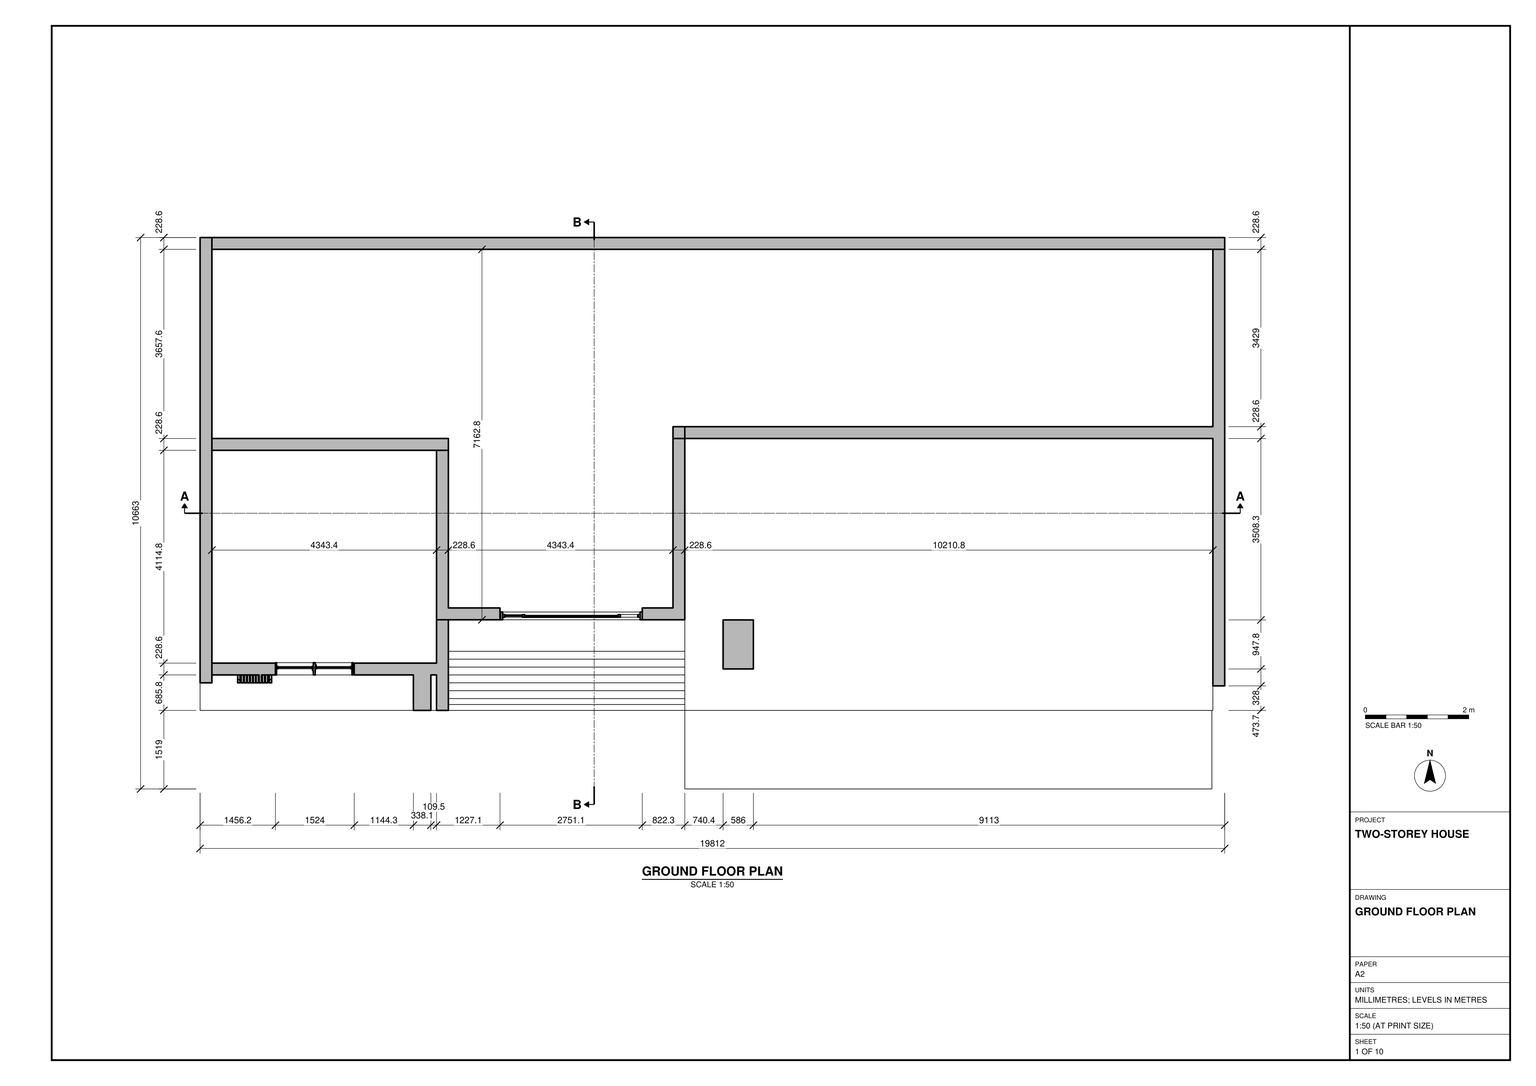
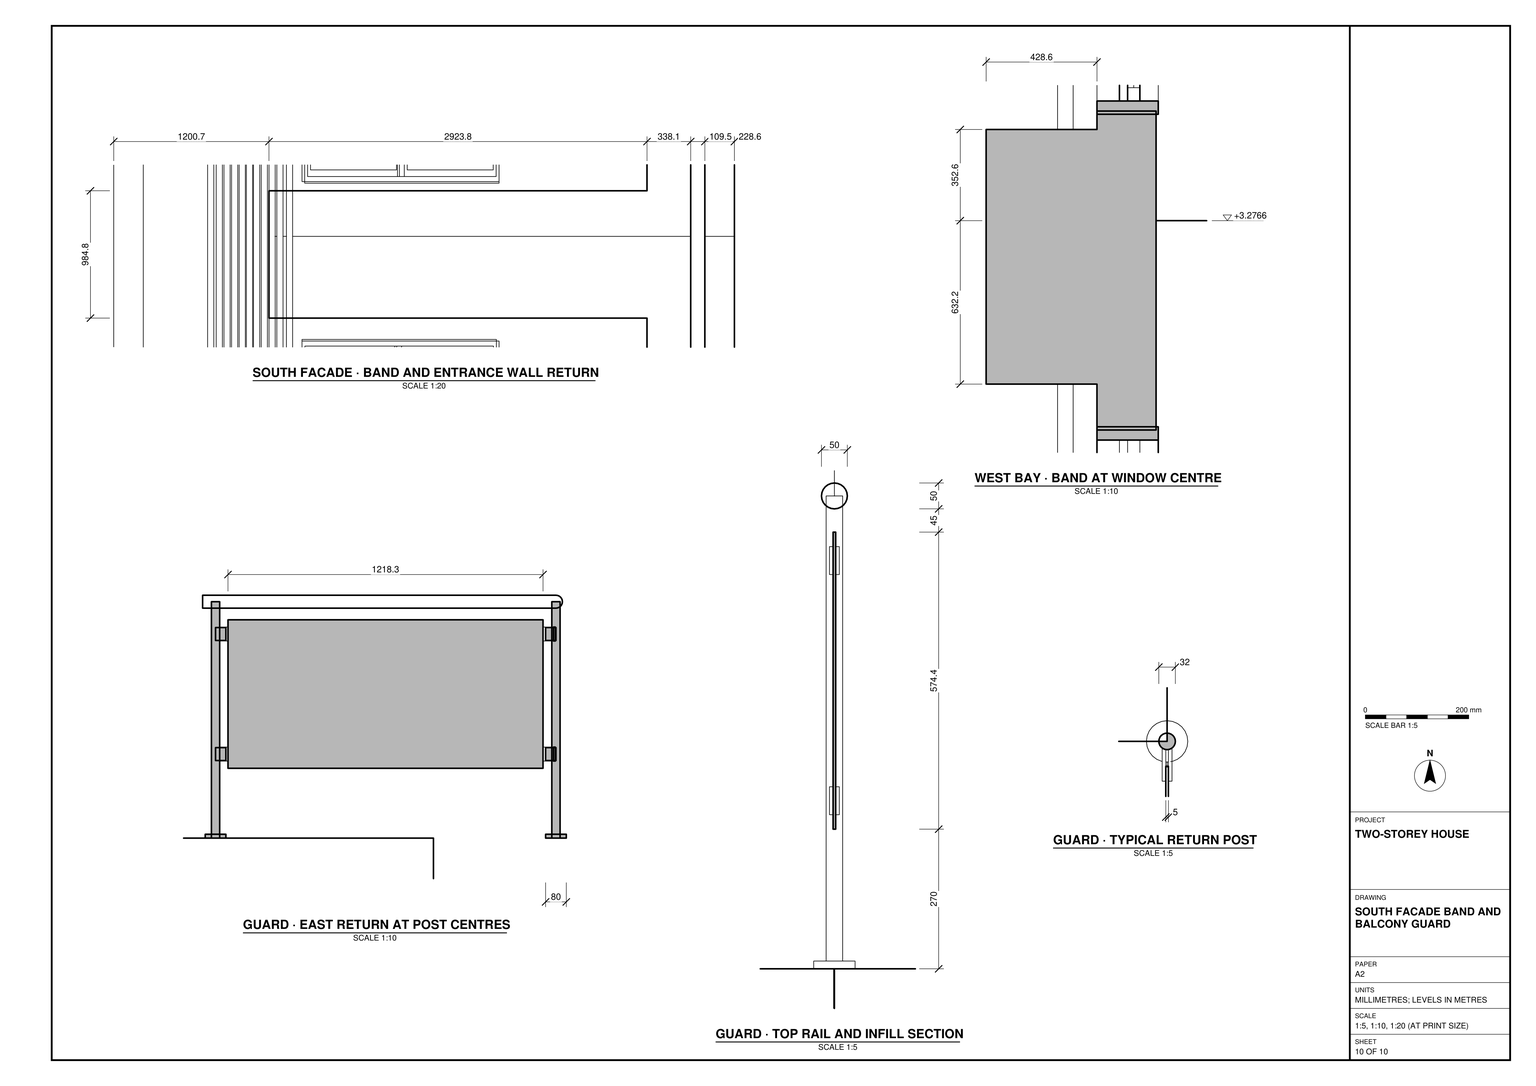
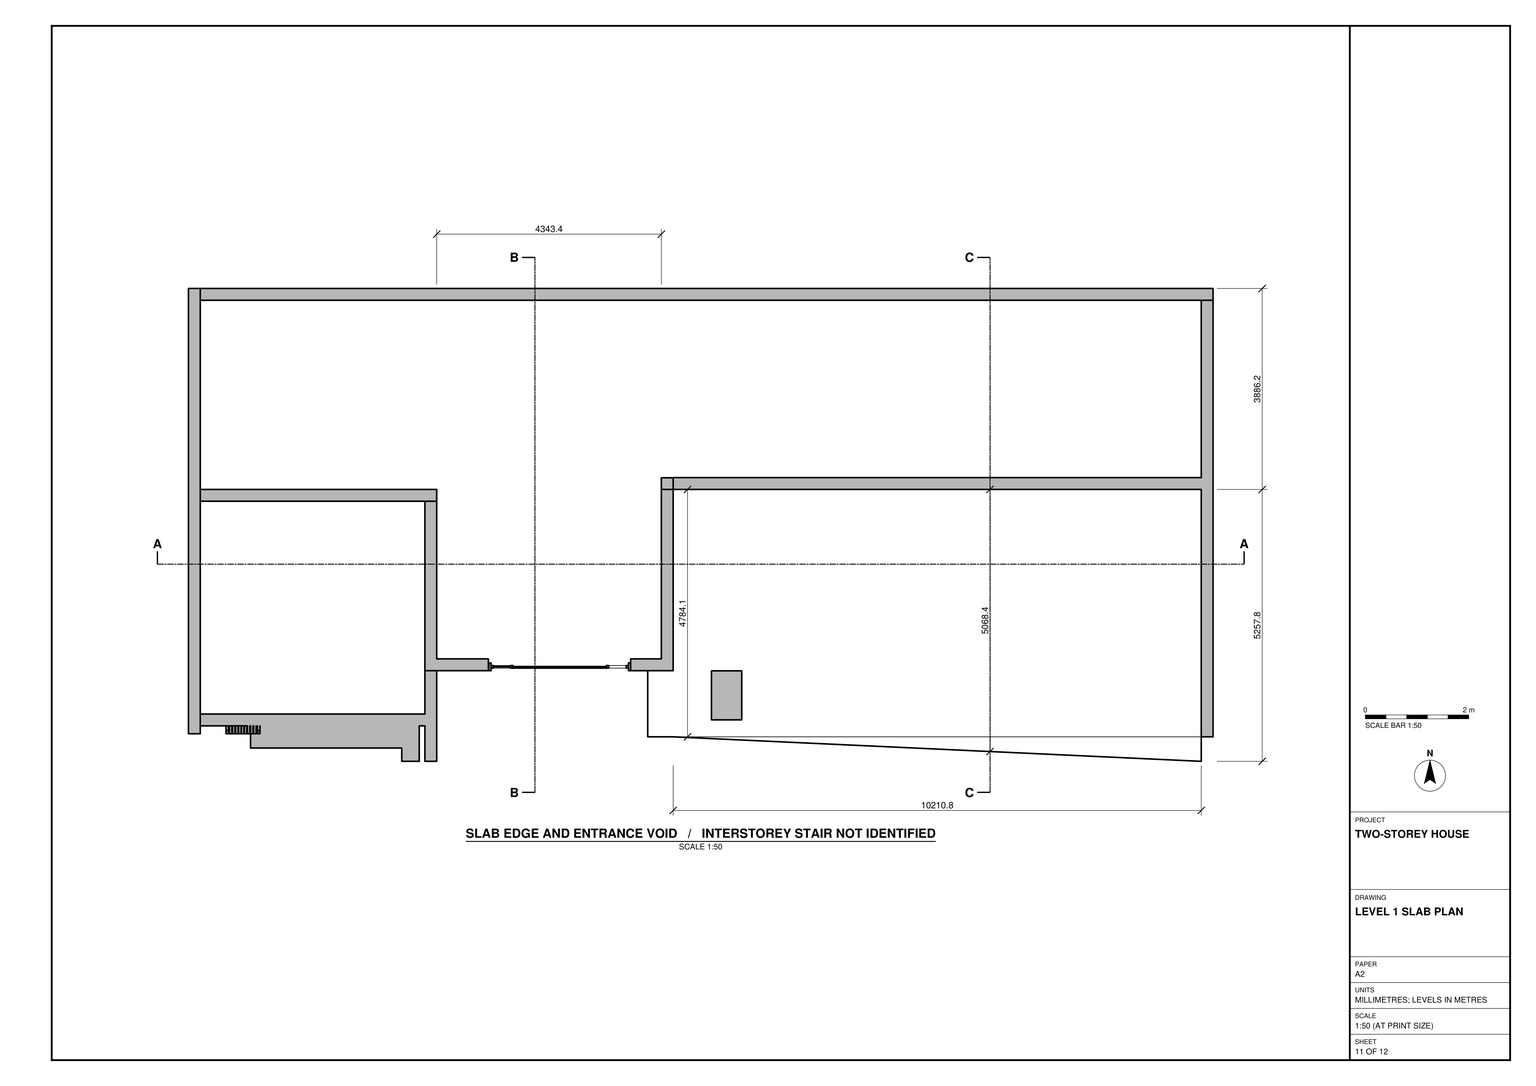
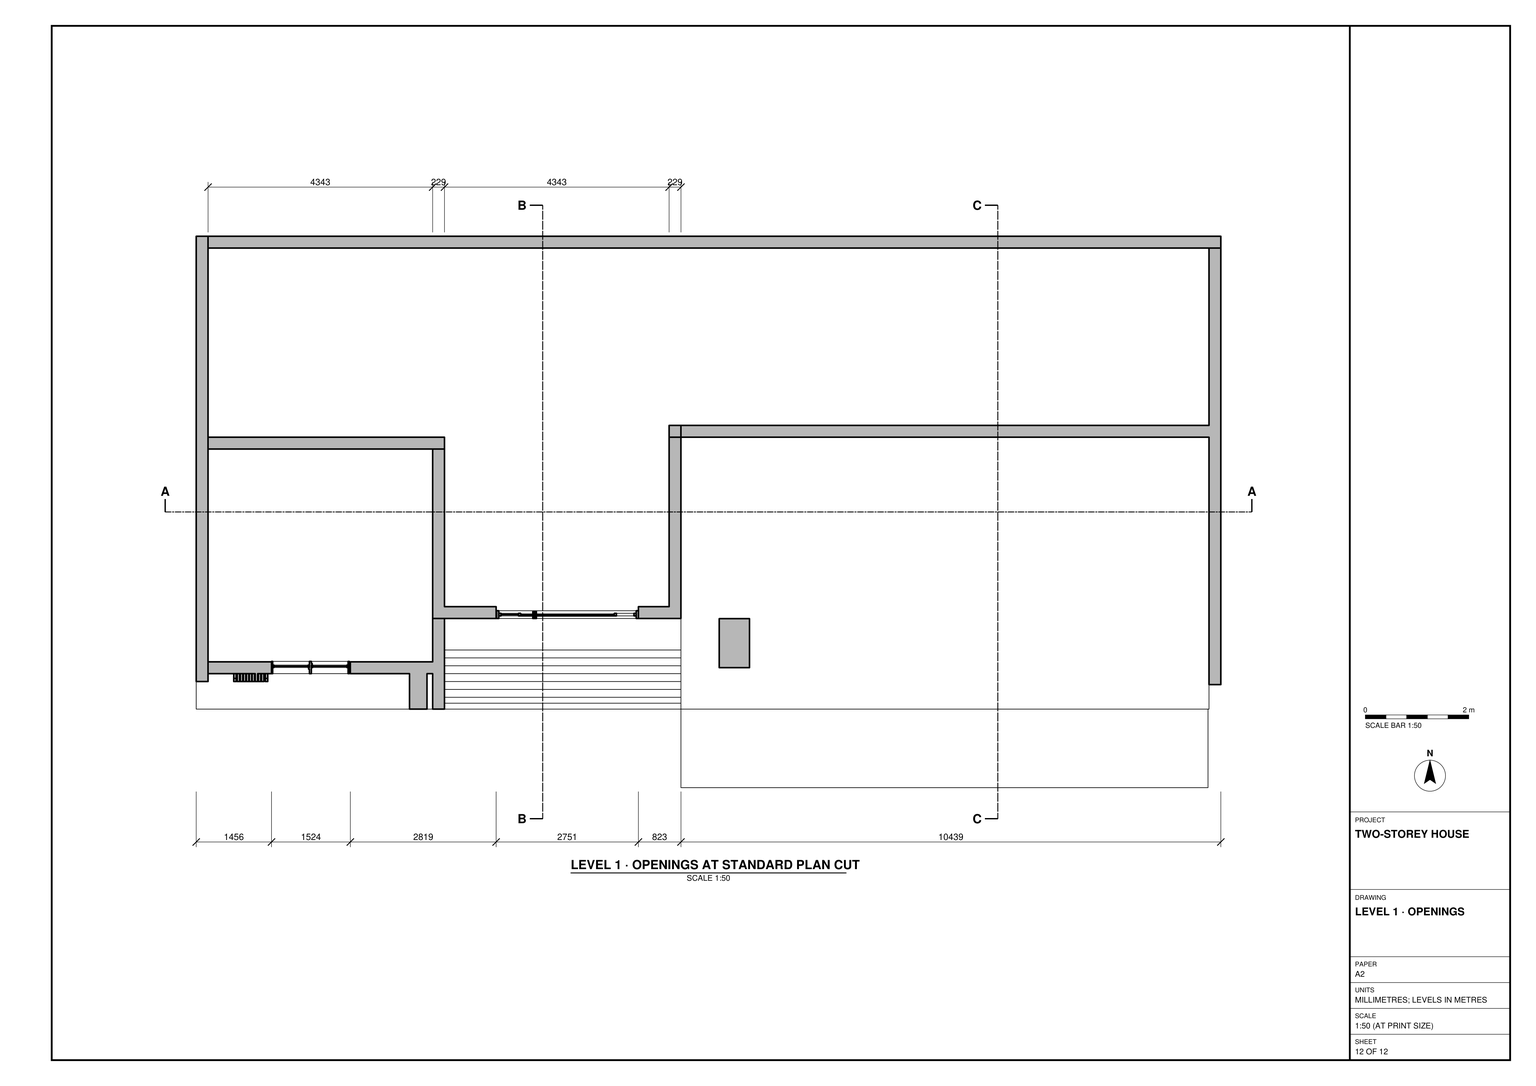
Build the house in SketchUp from task_files/diagram_01.pdf. Work in millimetres and orient the plan with the entrance on the south side. The overall model is 19812 mm wide from west to east, 10663.2 mm deep from north to south and 8074 mm high. Set the ground floor at 0 mm and the upper floor at +3276.6 mm.

Lay out the continuous north wall, the west bay, the central entrance bay and the wider east bay. Use the wall thicknesses shown, including the walls dimensioned at 228.6 mm. Fit the door and window units into their openings. Run the exterior steps across the central bay up to the entrance and place the rectangular pier to their east.

Use the slab plan to shape the upper floor around the entrance void and to set out the angled balcony edge over the east bay. Follow the sheets for the roof profile. Model the projecting horizontal band on the west bay where it meets the entrance wall return. Use the guard details to place the balcony posts, top rail and raised infill panels, including the return at the east end.

Include built-in joinery and main furniture only where shown. Decor and loose items may be any suitable library components. Keep the walls, slabs, roof and each furniture or joinery piece in separate groups or components, and use components for repeated parts. Save one SketchUp model as output_files/two_storey_house_with_a_recessed_entrance_and_balcony.skp.

# SketchUp Ruby script. Lengths in millimetres.
U = 1.mm
M = Sketchup.active_model
def pt(a) = Geom::Point3d.new(a.map { |v| v * U })
def face(e, loops, mat)
  f = e.add_face(loops[0].map { |a| pt(a) })
  loops[1..].each { |l| e.add_face(l.map { |a| pt(a) }).erase! }
  f.material = f.back_material = mat if mat
  f
end
# faces: each face lists its corners as indices into pts; further lists are holes
def faces(e, pts, list, mat = nil) = list.each { |f| face(e, (f[0].is_a?(Array) ? f : [f]).map { |l| l.map { |i| pts[i] } }, mat) }
# xy, xz, yz: faces in a plane at the given z, y or x. An outline is a flat list of corners, or four numbers for a rectangle; further outlines are holes
def ring(l) = l.size == 4 ? [[l[0], l[1]], [l[2], l[1]], [l[2], l[3]], [l[0], l[3]]] : l.each_slice(2).to_a
def flat(e, list, mat, &to3) = list.each { |f| face(e, (f[0].is_a?(Array) ? f : [f]).map { |l| ring(l).map { |u, v| to3.(u, v) } }, mat) }
def xy(e, z, list, mat = nil) = flat(e, list, mat) { |x, y| [x, y, z] }
def xz(e, y, list, mat = nil) = flat(e, list, mat) { |x, z| [x, y, z] }
def yz(e, x, list, mat = nil) = flat(e, list, mat) { |y, z| [x, y, z] }
def lines(e, pts, list) = list.each { |a, b| e.add_line(pt(pts[a]), pt(pts[b])) }
# prism: a flat outline (further loops are holes) pulled along v
def prism(e, loops, v, mat = nil)
  f = face(e, loops, mat); d = Geom::Vector3d.new(v.map { |x| x * U })
  f.pushpull(f.normal.samedirection?(d) ? d.length : -d.length)
end
def box(e, o, s, mat = nil) = prism(e, [[o, [o[0] + s[0], o[1], o[2]], [o[0] + s[0], o[1] + s[1], o[2]], [o[0], o[1] + s[1], o[2]]]], [0, 0, s[2]], mat)
def at(x, y, z, deg = 0) = Geom::Transformation.translation(pt([x, y, z])) * Geom::Transformation.rotation(ORIGIN, Z_AXIS, deg.degrees)
def axes(o, x, y, z) = Geom::Transformation.new([*x, 0, *y, 0, *z, 0, *pt(o).to_a, 1])
def part(name) = M.definitions.add(name)
# library, detail: a bought-in or finely detailed component or shape, given as its bounding box
def library(name, o, s) = part(name).tap { |d| box(d.entities, o, s) }
def detail(e, o, s) = box(e.add_group.entities, o, s)
def put(e, d, t, mat = nil) = e.add_instance(d, t).tap { |i| i.material = mat if mat }
def group(e, t, mat = nil) = e.add_group.tap { |g| g.transformation = t; g.material = mat if mat }.entities
root = M.entities
M.materials.add("Glass").color = [0, 0, 0]
M.materials["Glass"].alpha = 0.1
M.materials.add("Madeira").color = [179, 133, 92]
M.materials.add("Metal").color = [102, 102, 102]
M.materials.add("Teddy_Hair").color = [48, 28, 16]
M.materials.add("Teddy_Paper").color = [237, 237, 189]
M.materials.add("[Asphalt New]").color = [67, 60, 62]
M.materials.add("[Granite Dark Gray]").color = [69, 68, 68]
M.materials.add("[Stone Brushed Khaki]").color = [226, 197, 133]
M.materials.add("[Wood Cherry Original]").color = [152, 86, 42]
c1 = part("Component\#4")
prism(c1.entities,[[[19.7,7.4,-50],[18.7,5,-50],[17.1,2.9,-50],[15,1.3,-50],[12.6,0.3,-50],[10,0,-50],[7.4,0.3,-50],[5,1.3,-50],[2.9,2.9,-50],[1.3,5,-50],[0.3,7.4,-50],[0,10,-50],[0.3,12.6,-50],[1.3,15,-50],[2.9,17.1,-50],[5,18.7,-50],[7.4,19.7,-50],[10,20,-50],[12.6,19.7,-50],[15,18.7,-50],[17.1,17.1,-50],[18.7,15,-50],[19.7,12.6,-50],[20,10,-50]]],[0,0,40])
c2 = part("Group\#63")
box(c2.entities,[0,-10,0],[50,10,790])
box(c2.entities,[0,-30,0],[50,10,790])
put(c2.entities,c1,axes([14.8,-30,616],[1,0,0],[0,0,1],[0,-1,0]))
put(c2.entities,c1,axes([14.8,-30,154],[1,0,0],[0,0,1],[0,-1,0]))
c3 = part("Sidelight frame")
xy(c3.entities,0,[[0,0,300,50]])
xy(c3.entities,30,[[30,0,270,50]])
xy(c3.entities,498.6,[[30,0,270,50]])
xy(c3.entities,528.6,[[30,0,270,50]])
xy(c3.entities,997.1,[[30,0,270,50]])
xy(c3.entities,1027.1,[[30,0,270,50]])
xy(c3.entities,1495.7,[[30,0,270,50]])
xy(c3.entities,1525.7,[[30,0,270,50]])
xy(c3.entities,2024.2,[[30,0,270,50]])
xy(c3.entities,2054.2,[[0,0,300,50]])
xz(c3.entities,0,[[[0,0,300,2054.2],[30,30,270,2024.2]],[30,498.6,270,528.6],[30,997.1,270,1027.1],[30,1495.7,270,1525.7]])
xz(c3.entities,50,[[[0,0,300,2054.2],[30,1525.7,270,2024.2],[30,528.6,270,997.1],[30,30,270,498.6],[30,1027.1,270,1495.7]]])
yz(c3.entities,0,[[0,0,50,2054.2]])
yz(c3.entities,30,[[0,30,50,498.6],[0,528.6,50,997.1],[0,1027.1,50,1495.7],[0,1525.7,50,2024.2]])
yz(c3.entities,270,[[0,30,50,498.6],[0,528.6,50,997.1],[0,1027.1,50,1495.7],[0,1525.7,50,2024.2]])
yz(c3.entities,300,[[0,0,50,2054.2]])
c4 = part("Glass pane")
box(c4.entities,[0,0,0],[240,3,498.6])
c5 = part("Group\#37")
put(c5.entities,c3,axes([1753.4,-100,0],[1,0,0],[0,1,0],[0,0,1.02202]),"Madeira")
g1 = group(c5.entities,at(0,-150,0),"Madeira")
xy(g1,0,[[140,0,170,150],[2054.2,0,2084.2,150]])
xy(g1,2099.4,[[170,0,2054.2,150]])
xy(g1,2129.4,[[140,0,2084.2,150]])
xz(g1,0,[[140,0,170,0,170,2099.4,2054.2,2099.4,2054.2,0,2084.2,0,2084.2,2129.4,140,2129.4]],"Madeira")
xz(g1,150,[[140,0,140,2129.4,2084.2,2129.4,2084.2,0,2054.2,0,2054.2,2099.4,170,2099.4,170,0]])
yz(g1,140,[[0,0,150,2129.4]])
yz(g1,170,[[0,0,50,2099.4],[100,0,150,2099.4]])
yz(g1,2054.2,[[0,0,150,2099.4]])
yz(g1,2084.2,[[0,0,150,2129.4]])
p = [[170,150,0],[2054.2,150,0]]
lines(g1,p,[[0,1]])
g2 = group(c5.entities,at(471.6,-70,0),"Madeira")
box(g2,[1.8,-30,2],[1278,30,2097.4])
g3 = group(c5.entities,at(170,-100,0))
put(g3,c3,axes([0,0,0],[1,0,0],[0,1,0],[0,0,1.02202]),"Madeira")
put(g3,c4,axes([30,25,1019.1],[1,0,0],[0,1,0],[0,0,1.02202]),"Glass")
put(g3,c4,axes([30,25,0],[1,0,0],[0,1,0],[0,0,1.02202]),"Glass")
put(g3,c4,axes([30,25,1559.3],[1,0,0],[0,1,0],[0,0,1.02202]),"Glass")
put(g3,c4,axes([30,25,509.5],[1,0,0],[0,1,0],[0,0,1.02202]),"Glass")
c6 = part("Group\#70")
yz(c6.entities,0,[[0,0,885,1080]])
c7 = part("Group\#1")
g4 = group(c7.entities,at(45,30,30))
prism(g4,[[[0,0,0],[0,0,1140],[0,945,1140],[0,945,0]],[[0,30,1110],[0,30,30],[0,915,30],[0,915,1110]]],[30,0,0])
put(g4,c6,at(15,30,30),"Glass")
g5 = group(c7.entities,at(0,0,0))
xy(g5,0,[[0,0,150,2000]])
xy(g5,30,[[0,30,150,30,150,975,95,975,95,955,75,955,75,975,0,975],[75,955,95,955,95,975,150,975,150,1025,45,1025,45,1045,25,1045,25,1025,0,1025,0,975,75,975],[0,1025,25,1025,25,1045,45,1045,45,1025,150,1025,150,1970,0,1970]])
xy(g5,1170,[[0,30,0,975,75,975,75,955,95,955,95,975,150,975,150,30],[75,955,75,975,0,975,0,1025,25,1025,25,1045,45,1045,45,1025,150,1025,150,975,95,975,95,955],[0,1025,0,1970,150,1970,150,1025,45,1025,45,1045,25,1045,25,1025]])
xy(g5,1200,[[0,0,150,2000]])
xz(g5,0,[[0,0,150,1200]])
xz(g5,30,[[0,30,150,1170]])
xz(g5,955,[[75,30,95,1170]])
xz(g5,975,[[0,30,75,1170],[95,30,150,1170]])
xz(g5,1025,[[0,30,25,1170],[45,30,150,1170]])
xz(g5,1045,[[25,30,45,1170]])
xz(g5,1970,[[0,30,150,1170]])
xz(g5,2000,[[0,0,150,1200]])
yz(g5,0,[[[0,0,2000,1200],[30,30,1970,1170]],[975,30,1025,1170]])
yz(g5,25,[[1025,30,1045,1170]])
yz(g5,45,[[1025,30,1045,1170]])
yz(g5,75,[[955,30,975,1170]])
yz(g5,95,[[955,30,975,1170]])
yz(g5,150,[[[0,0,2000,1200],[30,30,1970,1170]],[975,30,1025,1170]])
g6 = group(c7.entities,at(45,1025,30))
prism(g6,[[[0,0,0],[0,0,1140],[0,945,1140],[0,945,0]],[[0,30,1110],[0,30,30],[0,915,30],[0,915,1110]]],[30,0,0])
put(g6,c6,at(15,30,30),"Glass")
c8 = library("Group\#5",[0,0,0],[80,1378.9,939.4])
c9 = library("Group\#6",[0,0,0],[10546.9,1406.4,939.4])
xy(root,-233.4,[[9372.6,0,19564.4,1519.2]])
xy(root,-228.6,[[0,1519.2,0,2052.6,228.6,2052.6,228.6,2205,726.1,2205,726.1,2052.6,774,2052.6,774,2205,792.5,2205,792.5,2052.6,840.4,2052.6,840.4,2205,852.4,2205,852.4,2052.6,900.3,2052.6,900.3,2205,911.3,2205,911.3,2052.6,959.2,2052.6,959.2,2205,970,2205,970,2052.6,1017.9,2052.6,1017.9,2205,1026.3,2205,1026.3,2052.6,1074.2,2052.6,1074.2,2205,1081.1,2205,1081.1,2052.6,1129,2052.6,1129,2205,1140.7,2205,1140.7,2052.6,1188.6,2052.6,1188.6,2205,1201,2205,1201,2052.6,1248.9,2052.6,1248.9,2205,1261.5,2205,1261.5,2052.6,1309.4,2052.6,1309.4,2205,1335.7,2205,1335.7,2052.6,1383.6,2052.6,1383.6,2205,4124.5,2205,4124.5,1519.2],[4124.5,1519.2,4124.5,2205,1188.6,2205,1188.6,2052.6,1140.7,2052.6,1140.7,2205,228.6,2205,228.6,2433.6,4572,2433.6,4572,3271.8,4800.6,3271.8,4800.6,1519.2,4572,1519.2,4572,2205,4462.5,2205,4462.5,1519.2],[4462.5,1519.2,4572,2205],[[4800.6,1519.2,4800.6,1747.8,9372.6,1747.8,9372.6,6777,19583.4,6777,19583.4,1519.2],[10112.8,2320.9,10698.6,3268.8]],[4800.6,1747.8,9372.6,3271.8],
  [19583.4,1992.9,19812,10434.6],[0,2052.6,228.6,10663.2],[10112.8,2320.9,10698.6,3268.8],[228.6,2433.6,4572,6548.4],[5799.1,3271.8,5799.1,3500.4,4800.6,3500.4,4800.6,6777,228.6,6777,228.6,10434.6,19583.4,10434.6,19583.4,7005.6,9144,7005.6,9144,3500.4,8550.3,3500.4,8550.3,3271.8],
  [4572,3271.8,4572,6548.4,4800.6,6548.4,4800.6,3500.4,5799.1,3500.4,5799.1,3271.8],[8550.3,3271.8,9372.6,3500.4],[9144,3500.4,9372.6,6777],[228.6,6548.4,4800.6,6777],[9372.6,6777,19581.8,7005.6]])
xy(root,-38.1,[[9144,3500.4,9372.6,6777]])
xy(root,0,[[0,1519.2,4124.5,1519.2,4124.5,2205,1383.6,2205,1383.6,2052.6,1335.7,2052.6,1335.7,2205,1309.4,2205,1309.4,2052.6,1261.5,2052.6,1261.5,2205,1248.9,2205,1248.9,2052.6,1201,2052.6,1201,2205,1188.6,2205,1188.6,2052.6,1140.7,2052.6,1140.7,2205,1129,2205,1129,2052.6,1081.1,2052.6,1081.1,2205,1074.2,2205,1074.2,2052.6,1026.3,2052.6,1026.3,2205,1017.9,2205,1017.9,2052.6,970,2052.6,970,2205,959.2,2205,959.2,2052.6,911.3,2052.6,911.3,2205,900.3,2205,900.3,2052.6,852.4,2052.6,852.4,2205,840.4,2205,840.4,2052.6,792.5,2052.6,792.5,2205,774,2205,774,2052.6,726.1,2052.6,726.1,2205,228.6,2205,228.6,2052.6,0,2052.6],[4124.5,1519.2,4462.5,1519.2,4462.5,2205,4572,2205,4572,1519.2,4800.6,1519.2,4800.6,3271.8,4572,3271.8,4572,2433.6,228.6,2433.6,228.6,2205,1140.7,2205,1140.7,2052.6,1188.6,2052.6,1188.6,2205,4124.5,2205],[4462.5,1519.2,4572,2205],[[9372.6,1519.2,19583.4,6777],[10112.8,2320.9,10698.6,3268.8]],[4800.6,1633.5,9372.6,1747.8],
  [0,2052.6,228.6,10663.2],[726.1,2052.6,774,2113],[1335.7,2052.6,1383.6,2113],[10112.8,2320.9,10698.6,3268.8],[4572,3271.8,5799.1,3271.8,5799.1,3500.4,4800.6,3500.4,4800.6,6548.4,4572,6548.4],
  [8550.3,3271.8,9372.6,3500.4],[9144,3500.4,9372.6,6777],[228.6,6548.4,4800.6,6777],[9372.6,6777,19581.8,7005.6],[19581.8,6777,19583.4,7005.6],
  [228.6,10434.6,19812,10663.2]])
xy(root,0,[[4800.6,1519.2,9372.6,1633.5]],"Teddy_Paper")
xy(root,254,[[4800.6,1900.2,9372.6,2052.6]])
xy(root,254,[[4800.6,1747.8,9372.6,1900.2]],"Teddy_Paper")
xy(root,423.9,[[1456.2,2205,2980.2,2433.6]])
xy(root,508,[[4800.6,2205,9372.6,2357.4]])
xy(root,508,[[4800.6,2052.6,9372.6,2205]],"Teddy_Paper")
xy(root,762,[[4800.6,2357.4,9372.6,2509.8]])
xy(root,762,[[4800.6,2509.8,9372.6,2662.2]],"Teddy_Paper")
xy(root,914.4,[[4800.6,2662.2,9372.6,3271.8]])
xy(root,2467,[[1456.2,2205,2980.2,2433.6]])
xy(root,2644.4,[[1200.7,1776.4,4124.5,2205]])
xy(root,2835.3,[[8880.5,1992.9,19583.4,1992.9,19583.4,6777,9372.6,6777,9372.6,3271.8,8880.5,3271.8]])
xy(root,3048,[[19583.4,1519.2,19583.4,1992.9,9372.6,1992.9],[9144,7002.5,9372.6,7005.6]])
xy(root,3276.6,[[[19583.4,1519.2,19583.4,3466.2,19427.1,3466.2,19427.1,6777,9372.6,6777,9372.6,3271.8,8880.5,3271.8,8880.5,1992.9,9372.6,1992.9],[10112.8,2320.9,10698.6,3268.8]],[19583.4,1992.9,19812,6777],[228.6,2433.6,4572,6548.4],[4572,3271.8,4800.6,6548.4],[19427.1,3466.2,19583.4,3785.3],
  [9144,3500.4,9372.6,6777],[19427.1,3785.3,19583.4,6777],[228.6,6548.4,4800.6,6777],[9144,6777,9372.6,7002.5],[9372.6,6777,19581.8,7005.6],
  [19581.8,6777,19583.4,7005.6],[19583.4,6777,19812,10434.6],[9144,7002.5,9372.6,7005.6],[228.6,10434.6,19812,10663.2]])
xy(root,3629.2,[[1200.7,1776.4,4124.5,2205]],"[Granite Dark Gray]")
xy(root,3700.5,[[1456.2,2205,2980.2,2433.6]])
xy(root,4104.4,[[12655.7,6777,16238.7,7005.6]])
xy(root,5743.6,[[1456.2,2205,2980.2,2433.6]])
xy(root,5787.2,[[12655.7,6777,16238.7,7005.6]])
xy(root,5799.1,[[4800.6,1519.2,4800.6,3271.8,5799.1,3271.8,5799.1,3500.4,4800.6,3500.4,4800.6,6777,228.6,6777,228.6,10434.6,19583.4,10434.6,19583.4,7005.6,9144,7005.6,9144,3500.4,8550.3,3500.4,8550.3,3271.8,9372.6,3271.8,9372.6,6777,11168.5,6777,11168.5,1519.2]])
xy(root,6007.3,[[228.6,2052.6,726.1,2205]])
xy(root,6025,[[1383.6,2052.6,4124.5,2205]])
xy(root,6165.6,[[4572,1519.2,11168.5,2205]])
xy(root,6283.8,[[4462.5,1519.2,11168.5,2205]])
xy(root,6308.7,[[10112.8,2320.9,10698.6,3268.8]])
xy(root,6324.6,[[11669.7,3323.8,11971.9,6275.8],[12417.8,3323.8,12637.2,6275.8],[13079.9,3323.8,13329.7,6275.8],[13749.4,3323.8,13930.1,6275.8],[14410.6,3323.8,14614.6,6275.8],
  [15078.8,3323.8,15252,6275.8],[15735.8,3323.8,15895.9,6275.8],[16393.2,3323.8,16483,6275.8],[16958.6,3323.8,17042.9,6275.8],[17549.8,3323.8,17662.9,6275.8],
  [18112.5,3323.8,18183.2,6275.8],[18665,3323.8,18925.9,6275.8],[19427.1,3785.3,19583.4,6777],[9144,7002.5,9372.6,7005.6]])
xy(root,6324.6,[[[11168.5,2728.9,11168.5,6777,19427.1,6777,19427.1,3785.3,19583.4,3785.3,19583.4,2728.9],[11669.7,3323.8,18925.9,6275.8]]],"[Asphalt New]")
xy(root,6340.5,[[19427.1,3466.2,19583.4,3785.3]])
xy(root,6553.2,[[0,2052.6,228.6,10663.2],[228.6,2433.6,4572,6548.4],[4800.6,3271.8,5799.1,3283],[8550.3,3271.8,9372.6,3500.4],[4800.6,3283,5799.1,3500.4],
  [9144,3500.4,9372.6,6777],[228.6,6548.4,4800.6,6777],[9144,6777,9372.6,7002.5],[9372.6,6777,19812,6777,19812,10434.6,19583.4,10434.6,19583.4,7005.6,9372.6,7005.6],[228.6,10434.6,19812,10663.2]])
xy(root,6608.8,[[4572,2205,4800.6,3271.8],[4572,3271.8,4800.6,6548.4],[4800.6,4915.7,9144,4915.7,9144,7002.5,9372.6,7002.5,9372.6,7005.6,19583.4,7005.6,19583.4,10434.6,228.6,10434.6,228.6,6777,4800.6,6777]])
xy(root,6608.8,[[[4124.5,1519.2,11168.5,1519.2,11168.5,2728.9,19583.4,2728.9,19583.4,6777,9372.6,6777,9372.6,3271.8,8550.3,3271.8,8550.3,3500.4,4800.6,3500.4,4800.6,3283,5799.1,3283,5799.1,3271.8,4800.6,3271.8,4800.6,2205,4124.5,2205],[17042.9,3323.8,17549.8,6275.8],[15895.9,3323.8,16393.2,6275.8],[15252,3323.8,15735.8,6275.8],[18183.2,3323.8,18665,6275.8],[13930.1,3323.8,14410.6,6275.8],[16483,3323.8,16958.6,6275.8],[14614.6,3323.8,15078.8,6275.8],[17662.9,3323.8,18112.5,6275.8],[11971.9,3323.8,12417.8,6275.8],[12637.2,3323.8,13079.9,6275.8],[13329.7,3323.8,13749.4,6275.8]]],"Metal")
xy(root,6640.5,[[228.6,2052.6,726.1,2052.6,726.1,2333.6,774,2333.6,774,2205,792.5,2205,792.5,2333.6,840.4,2333.6,840.4,2205,852.4,2205,852.4,2333.6,900.3,2333.6,900.3,2205,911.3,2205,911.3,2333.6,959.2,2333.6,959.2,2205,970,2205,970,2333.6,1017.9,2333.6,1017.9,2205,1026.3,2205,1026.3,2333.6,1074.2,2333.6,1074.2,2205,1081.1,2205,1081.1,2333.6,1129,2333.6,1129,2205,1140.7,2205,1140.7,2333.6,1188.6,2333.6,1188.6,2205,1201,2205,1201,2333.6,1248.9,2333.6,1248.9,2205,1261.5,2205,1261.5,2333.6,1309.4,2333.6,1309.4,2205,1335.7,2205,1335.7,2333.6,1383.6,2333.6,1383.6,2052.6,4124.5,2052.6,4124.5,2205,4572,2205,4572,2433.6,228.6,2433.6]])
xy(root,6640.5,[[726.1,2052.6,774,2113],[792.5,2052.6,840.4,2205],[852.4,2052.6,900.3,2205],[911.3,2052.6,959.2,2205],[970,2052.6,1017.9,2205],
  [1026.3,2052.6,1074.2,2205],[1081.1,2052.6,1129,2205],[1140.7,2052.6,1188.6,2333.6],[1201,2052.6,1248.9,2205],[1261.5,2052.6,1309.4,2205],
  [1335.7,2052.6,1383.6,2113],[726.1,2113,774,2205],[1335.7,2113,1383.6,2205],[726.1,2205,774,2333.6],[792.5,2205,840.4,2333.6],
  [852.4,2205,900.3,2333.6],[911.3,2205,959.2,2333.6],[970,2205,1017.9,2333.6],[1026.3,2205,1074.2,2333.6],[1081.1,2205,1129,2333.6],
  [1201,2205,1248.9,2333.6],[1261.5,2205,1309.4,2333.6],[1335.7,2205,1383.6,2333.6]],"[Asphalt New]")
xy(root,7739.1,[[3984.6,1285.9,9144,8222.5]],"Madeira")
xy(root,7840.7,[[3984.6,1285.9,9144,8222.5]])
xz(root,1285.9,[[3984.6,7739.1,9144,7840.7]])
xz(root,1519.2,[[9372.6,-233.4,19564.4,-228.6],[0,-228.6,4124.5,0],[4124.5,-228.6,4462.5,0],[4462.5,-228.6,4572,0],[4572,-228.6,4800.6,0],
  [4800.6,-228.6,9372.6,0],[9372.6,-228.6,19564.4,0],[19564.4,-228.6,19583.4,0]])
xz(root,1519.2,[[4124.5,0,4462.5,0,4462.5,6283.8,11168.5,6283.8,11168.5,6608.8,4124.5,6608.8],[4572,0,4800.6,0,4800.6,5799.1,11168.5,5799.1,11168.5,6165.6,4572,6165.6]],"Metal")
xz(root,1747.8,[[4800.6,-228.6,9372.6,0],[4800.6,0,9372.6,254]])
xz(root,1776.4,[[1200.7,2644.4,4124.5,3629.2]],"[Granite Dark Gray]")
xz(root,1992.9,[[9372.6,2835.3,19583.4,3048]])
xz(root,1992.9,[[8880.5,2835.3,9372.6,3276.6]],"Teddy_Hair")
xz(root,1992.9,[[19583.4,-228.6,19812,3276.6]],"[Granite Dark Gray]")
xz(root,2052.6,[[0,-228.6,228.6,0],[726.1,-228.6,774,0],[1140.7,-228.6,1188.6,0],[1335.7,-228.6,1383.6,0],[4800.6,254,9372.6,508]])
xz(root,2052.6,[[0,0,0,6553.2,228.6,6553.2,228.6,6640.5,726.1,6640.5,726.1,6007.3,228.6,6007.3,228.6,0],[1383.6,6025,4124.5,6640.5]],"Metal")
xz(root,2052.6,[[792.5,-228.6,840.4,6640.5],[852.4,-228.6,900.3,6640.5],[911.3,-228.6,959.2,6640.5],[970,-228.6,1017.9,6640.5],[1026.3,-228.6,1074.2,6640.5],
  [1081.1,-228.6,1129,6640.5],[1201,-228.6,1248.9,6640.5],[1261.5,-228.6,1309.4,6640.5],[726.1,0,774,6640.5],[1140.7,0,1188.6,6640.5],
  [1335.7,0,1383.6,6640.5]],"[Asphalt New]")
xz(root,2113,[[726.1,0,774,6640.5],[1335.7,0,1383.6,6640.5]])
xz(root,2205,[[228.6,-228.6,726.1,0],[726.1,-228.6,774,0],[774,-228.6,792.5,0],[792.5,-228.6,840.4,0],[840.4,-228.6,852.4,0],
  [852.4,-228.6,900.3,0],[900.3,-228.6,911.3,0],[911.3,-228.6,959.2,0],[959.2,-228.6,970,0],[970,-228.6,1017.9,0],
  [1017.9,-228.6,1026.3,0],[1026.3,-228.6,1074.2,0],[1074.2,-228.6,1081.1,0],[1081.1,-228.6,1129,0],[1129,-228.6,1140.7,0],
  [1188.6,-228.6,1201,0],[1201,-228.6,1248.9,0],[1248.9,-228.6,1261.5,0],[1261.5,-228.6,1309.4,0],[1309.4,-228.6,1335.7,0],
  [1335.7,-228.6,1383.6,0],[1383.6,-228.6,4124.5,0],[4462.5,-228.6,4572,0],[726.1,0,774,6640.5],[774,0,792.5,6640.5],
  [792.5,0,840.4,6640.5],[840.4,0,852.4,6640.5],[852.4,0,900.3,6640.5],[900.3,0,911.3,6640.5],[911.3,0,959.2,6640.5],
  [959.2,0,970,6640.5],[970,0,1017.9,6640.5],[1017.9,0,1026.3,6640.5],[1026.3,0,1074.2,6640.5],[1074.2,0,1081.1,6640.5],
  [1081.1,0,1129,6640.5],[1129,0,1140.7,6640.5],[1188.6,0,1201,0,1201,2644.4,1200.7,2644.4,1200.7,3629.2,1201,3629.2,1201,6640.5,1188.6,6640.5],[1201,0,1248.9,2644.4],[1248.9,0,1261.5,2644.4],
  [1261.5,0,1309.4,2644.4],[1309.4,0,1335.7,2644.4],[1335.7,0,1383.6,2644.4],[1201,3629.2,1248.9,6640.5],[1248.9,3629.2,1261.5,6640.5],
  [1261.5,3629.2,1309.4,6640.5],[1309.4,3629.2,1335.7,6640.5],[1335.7,3629.2,1383.6,6640.5],[4124.5,6324.6,4572,6608.8],[4572,6324.6,4800.6,6608.8],
  [4124.5,6608.8,4572,6640.5]])
xz(root,2205,[[4462.5,0,4572,0,4572,6165.6,4800.6,6165.6,4800.6,6283.8,4462.5,6283.8],[4800.6,6165.6,11168.5,6283.8]],"Teddy_Paper")
xz(root,2205,[[228.6,0,726.1,6007.3],[[1383.6,0,4124.5,2644.4],[1456.2,423.9,2980.2,2467]],[[1383.6,3629.2,4124.5,6025],[1456.2,3700.5,2980.2,5743.6]]],"[Wood Cherry Original]")
xz(root,2320.9,[[10112.8,-228.6,10698.6,0],[10112.8,0,10698.6,3276.6],[10112.8,3276.6,10698.6,6308.7]])
xz(root,2357.4,[[4800.6,508,9372.6,762]])
xz(root,2433.6,[[228.6,-228.6,4572,0],[[228.6,0,4572,3276.6],[1456.2,423.9,2980.2,2467]],[[228.6,3276.6,4572,6553.2],[1456.2,3700.5,2980.2,5743.6]],[228.6,6553.2,4572,6640.5]])
xz(root,2662.2,[[4800.6,762,9372.6,914.4]])
xz(root,2728.9,[[11168.5,6324.6,19583.4,6608.8]],"[Asphalt New]")
xz(root,3268.8,[[10112.8,-228.6,10698.6,0],[10112.8,0,10698.6,3276.6],[10112.8,3276.6,10698.6,6308.7]])
xz(root,3271.8,[[4572,-228.6,4800.6,0],[4800.6,-228.6,5799.1,0],[5799.1,-228.6,8550.3,914.4],[8550.3,-228.6,9372.6,0],[4572,0,4800.6,3276.6],
  [4800.6,0,5799.1,914.4],[8550.3,0,9372.6,914.4],[8880.5,2835.3,9372.6,3276.6],[4572,3276.6,4800.6,6608.8],[4800.6,5799.1,5799.1,6553.2],
  [8550.3,5799.1,9372.6,6553.2],[4800.6,6553.2,5799.1,6608.8],[8550.3,6553.2,9372.6,6608.8]])
xz(root,3271.8,[[4800.6,914.4,5799.1,5799.1],[8550.3,914.4,9372.6,914.4,9372.6,2835.3,8880.5,2835.3,8880.5,3276.6,9372.6,3276.6,9372.6,5799.1,8550.3,5799.1]],"[Stone Brushed Khaki]")
xz(root,3283,[[4800.6,6553.2,5799.1,6608.8]])
xz(root,3323.8,[[11971.9,6324.6,12417.8,6608.8],[12637.2,6324.6,13079.9,6608.8],[13329.7,6324.6,13749.4,6608.8],[13930.1,6324.6,14410.6,6608.8],[14614.6,6324.6,15078.8,6608.8],
  [15252,6324.6,15735.8,6608.8],[15895.9,6324.6,16393.2,6608.8],[16483,6324.6,16958.6,6608.8],[17042.9,6324.6,17549.8,6608.8],[17662.9,6324.6,18112.5,6608.8],
  [18183.2,6324.6,18665,6608.8]])
xz(root,3500.4,[[4800.6,-228.6,5799.1,0],[8550.3,-228.6,9144,0],[9144,-228.6,9372.6,-38.1],[9144,-38.1,9372.6,0],[4800.6,0,5799.1,3048],
  [8550.3,0,9144,3048],[4800.6,3048,5799.1,3276.6],[8550.3,3048,9144,3276.6],[4800.6,3276.6,5799.1,5799.1],[8550.3,3276.6,9144,5799.1],
  [4800.6,5799.1,5799.1,6553.2],[8550.3,5799.1,9144,6553.2]])
xz(root,3785.3,[[19427.1,6324.6,19583.4,6340.5]])
xz(root,6275.8,[[11971.9,6324.6,12417.8,6608.8],[12637.2,6324.6,13079.9,6608.8],[13329.7,6324.6,13749.4,6608.8],[13930.1,6324.6,14410.6,6608.8],[14614.6,6324.6,15078.8,6608.8],
  [15252,6324.6,15735.8,6608.8],[15895.9,6324.6,16393.2,6608.8],[16483,6324.6,16958.6,6608.8],[17042.9,6324.6,17549.8,6608.8],[17662.9,6324.6,18112.5,6608.8],
  [18183.2,6324.6,18665,6608.8]])
xz(root,6548.4,[[228.6,-228.6,4572,0],[4572,-228.6,4800.6,0],[228.6,0,4572,3276.6],[4572,0,4800.6,3276.6],[228.6,3276.6,4572,6553.2],
  [4572,3276.6,4800.6,6553.2],[4572,6553.2,4800.6,6608.8]])
xz(root,6777,[[228.6,-228.6,4800.6,0],[9144,-228.6,9372.6,-38.1],[9372.6,-228.6,19581.8,0],[19581.8,-228.6,19583.4,0],[9144,-38.1,9372.6,0],
  [228.6,0,4800.6,3048],[9144,0,9372.6,3276.6],[9372.6,0,19581.8,2835.3],[19581.8,0,19583.4,2835.3],[9372.6,2835.3,19581.8,3276.6],
  [19581.8,2835.3,19583.4,3276.6],[228.6,3048,4800.6,3276.6],[228.6,3276.6,4800.6,5799.1],[9144,3276.6,9372.6,6553.2],[228.6,5799.1,4800.6,6553.2],
  [9372.6,5799.1,9372.6,6553.2,19581.8,6553.2,19581.8,6324.6,11168.5,6324.6,11168.5,5799.1],[19581.8,6324.6,19583.4,6553.2],[228.6,6553.2,4800.6,6608.8],[9372.6,6553.2,19581.8,6608.8],[19581.8,6553.2,19583.4,6608.8]])
xz(root,6777,[[[9372.6,3276.6,19812,3276.6,19812,6553.2,19583.4,6553.2,19583.4,6324.6,11168.5,6324.6,11168.5,5799.1,9372.6,5799.1],[12655.7,4104.4,16238.7,5787.2]]],"[Stone Brushed Khaki]")
xz(root,7002.5,[[9144,3048,9372.6,3276.6],[9144,6324.6,9372.6,6553.2],[9144,6553.2,9372.6,6608.8]])
xz(root,7005.6,[[9144,-228.6,9372.6,3048],[9372.6,-228.6,19581.8,0],[19581.8,-228.6,19583.4,0],[9372.6,0,19581.8,3048],[19581.8,0,19583.4,3048],
  [9372.6,3048,19581.8,3276.6],[19581.8,3048,19583.4,3276.6],[9144,3276.6,9372.6,5799.1],[[9372.6,3276.6,19581.8,5799.1],[12655.7,4104.4,16238.7,5787.2]],[19581.8,3276.6,19583.4,5799.1],
  [9144,5799.1,9372.6,6324.6],[9372.6,5799.1,19581.8,6553.2],[19581.8,5799.1,19583.4,6553.2],[9372.6,6553.2,19581.8,6608.8],[19581.8,6553.2,19583.4,6608.8]])
xz(root,8222.5,[[3984.6,7739.1,9144,7840.7]])
xz(root,10434.6,[[228.6,-228.6,19583.4,0],[19583.4,-228.6,19812,0],[228.6,0,19583.4,3048],[19583.4,0,19812,3276.6],[228.6,3048,19583.4,3276.6],
  [228.6,3276.6,19583.4,5799.1],[19583.4,3276.6,19812,6553.2],[228.6,5799.1,19583.4,6553.2],[228.6,6553.2,19583.4,6608.8]])
xz(root,10663.2,[[0,-228.6,228.6,0],[0,0,228.6,3276.6],[228.6,0,19812,3276.6],[0,3276.6,228.6,6553.2],[228.6,3276.6,19812,6553.2]])
yz(root,0,[[1519.2,-228.6,2052.6,0],[2052.6,-228.6,10663.2,0],[2052.6,0,10663.2,3276.6],[2052.6,3276.6,10663.2,6553.2]])
yz(root,228.6,[[2052.6,-228.6,2205,0],[2205,-228.6,2433.6,0],[2433.6,-228.6,6548.4,0],[6548.4,-228.6,6777,0],[6777,-228.6,10434.6,0],
  [10434.6,-228.6,10663.2,0],[2052.6,0,2205,3276.6],[2205,0,2433.6,3276.6],[2433.6,0,6548.4,3276.6],[6548.4,0,6777,3276.6],
  [6777,0,10434.6,3048],[10434.6,0,10663.2,3276.6],[6777,3048,10434.6,3276.6],[2052.6,3276.6,2205,6007.3],[2433.6,3276.6,6548.4,6553.2],
  [6548.4,3276.6,6777,6553.2],[6777,3276.6,10434.6,5799.1],[10434.6,3276.6,10663.2,6553.2],[6777,5799.1,10434.6,6553.2],[2052.6,6553.2,2433.6,6640.5],
  [6777,6553.2,10434.6,6608.8]])
yz(root,726.1,[[2052.6,-228.6,2113,0],[2113,-228.6,2205,0],[2052.6,0,2113,6007.3],[2113,0,2205,6007.3],[2052.6,6007.3,2113,6640.5],
  [2113,6007.3,2205,6640.5],[2205,6553.2,2333.6,6640.5]])
yz(root,774,[[2052.6,-228.6,2113,0],[2113,-228.6,2205,0],[2052.6,0,2113,6640.5],[2113,0,2205,6640.5],[2205,6553.2,2333.6,6640.5]])
yz(root,792.5,[[2052.6,-228.6,2205,0],[2205,6553.2,2333.6,6640.5]])
yz(root,792.5,[[2052.6,0,2205,6640.5]],"[Wood Cherry Original]")
yz(root,840.4,[[2052.6,-228.6,2205,0],[2052.6,0,2205,6640.5],[2205,6553.2,2333.6,6640.5]])
yz(root,852.4,[[2052.6,-228.6,2205,0],[2205,6553.2,2333.6,6640.5]])
yz(root,852.4,[[2052.6,0,2205,6640.5]],"[Wood Cherry Original]")
yz(root,900.3,[[2052.6,-228.6,2205,0],[2205,6553.2,2333.6,6640.5]])
yz(root,900.3,[[2052.6,0,2205,6640.5]],"[Wood Cherry Original]")
yz(root,911.3,[[2052.6,-228.6,2205,0],[2205,6553.2,2333.6,6640.5]])
yz(root,911.3,[[2052.6,0,2205,6640.5]],"[Asphalt New]")
yz(root,959.2,[[2052.6,-228.6,2205,0],[2205,6553.2,2333.6,6640.5]])
yz(root,959.2,[[2052.6,0,2205,6640.5]],"[Wood Cherry Original]")
yz(root,970,[[2052.6,-228.6,2205,0],[2205,6553.2,2333.6,6640.5]])
yz(root,970,[[2052.6,0,2205,6640.5]],"[Wood Cherry Original]")
yz(root,1017.9,[[2052.6,-228.6,2205,0],[2205,6553.2,2333.6,6640.5]])
yz(root,1017.9,[[2052.6,0,2205,6640.5]],"[Wood Cherry Original]")
yz(root,1026.3,[[2052.6,-228.6,2205,0],[2205,6553.2,2333.6,6640.5]])
yz(root,1026.3,[[2052.6,0,2205,6640.5]],"[Wood Cherry Original]")
yz(root,1074.2,[[2052.6,-228.6,2205,0],[2205,6553.2,2333.6,6640.5]])
yz(root,1074.2,[[2052.6,0,2205,6640.5]],"[Wood Cherry Original]")
yz(root,1081.1,[[2052.6,-228.6,2205,0],[2052.6,0,2205,6640.5],[2205,6553.2,2333.6,6640.5]])
yz(root,1129,[[2052.6,-228.6,2205,0],[2205,6553.2,2333.6,6640.5]])
yz(root,1129,[[2052.6,0,2205,6640.5]],"[Wood Cherry Original]")
yz(root,1140.7,[[2052.6,-228.6,2205,0]])
yz(root,1140.7,[[2052.6,0,2205,6640.5]],"[Wood Cherry Original]")
yz(root,1188.6,[[2052.6,-228.6,2205,0]])
yz(root,1188.6,[[2052.6,0,2205,6640.5]],"[Wood Cherry Original]")
yz(root,1200.7,[[1776.4,2644.4,2205,3629.2]],"[Granite Dark Gray]")
yz(root,1201,[[2052.6,-228.6,2205,0],[2205,6553.2,2333.6,6640.5]])
yz(root,1201,[[2052.6,0,2205,6640.5]],"[Wood Cherry Original]")
yz(root,1248.9,[[2052.6,-228.6,2205,0],[2205,6553.2,2333.6,6640.5]])
yz(root,1248.9,[[2052.6,0,2205,6640.5]],"[Wood Cherry Original]")
yz(root,1261.5,[[2052.6,-228.6,2205,0],[2205,6553.2,2333.6,6640.5]])
yz(root,1261.5,[[2052.6,0,2205,6640.5]],"[Wood Cherry Original]")
yz(root,1309.4,[[2052.6,-228.6,2205,0],[2205,6553.2,2333.6,6640.5]])
yz(root,1309.4,[[2052.6,0,2205,6640.5]],"[Wood Cherry Original]")
yz(root,1335.7,[[2052.6,-228.6,2113,0],[2113,-228.6,2205,0],[2205,6553.2,2333.6,6640.5]])
yz(root,1335.7,[[2052.6,0,2113,6640.5],[2113,0,2205,6640.5]],"[Wood Cherry Original]")
yz(root,1383.6,[[2052.6,-228.6,2113,0],[2113,-228.6,2205,0],[2052.6,0,2113,6025],[2113,0,2205,6025],[2052.6,6025,2113,6640.5],
  [2113,6025,2205,6640.5],[2205,6553.2,2333.6,6640.5]])
yz(root,1456.2,[[2205,423.9,2433.6,2467],[2205,3700.5,2433.6,5743.6]])
yz(root,2980.2,[[2205,423.9,2433.6,2467],[2205,3700.5,2433.6,5743.6]])
yz(root,3984.6,[[1285.9,7739.1,8222.5,7840.7]])
yz(root,4124.5,[[1519.2,-228.6,2205,0],[2052.6,6324.6,2205,6608.8],[2052.6,6608.8,2205,6640.5]])
yz(root,4124.5,[[1519.2,0,1519.2,6608.8,2052.6,6608.8,2052.6,6025,2205,6025,2205,3629.2,1776.4,3629.2,1776.4,2644.4,2205,2644.4,2205,0]],"Metal")
yz(root,4462.5,[[1519.2,-228.6,2205,0],[1519.2,0,2205,6283.8]])
yz(root,4572,[[1519.2,-228.6,2205,0],[2433.6,-228.6,3271.8,0],[3271.8,-228.6,6548.4,0],[1519.2,0,2205,6165.6],[2433.6,0,3271.8,3276.6],
  [3271.8,0,6548.4,3276.6],[2433.6,3276.6,3271.8,6553.2],[3271.8,3276.6,6548.4,6553.2],[2433.6,6553.2,3271.8,6608.8],[3271.8,6553.2,6548.4,6608.8],
  [2205,6608.8,2433.6,6640.5]])
yz(root,4800.6,[[1519.2,-228.6,1747.8,0],[1747.8,-228.6,3271.8,0],[3500.4,-228.6,6548.4,0],[6548.4,-228.6,6777,0],[1519.2,0,1747.8,254],
  [1747.8,0,3271.8,0,3271.8,914.4,2662.2,914.4,2662.2,762,2357.4,762,2357.4,508,2052.6,508,2052.6,254,1747.8,254],[3500.4,0,6548.4,3048],[6548.4,0,6777,3048],[1519.2,254,2052.6,508],[1519.2,508,2357.4,508,2357.4,762,2662.2,762,2662.2,914.4,3271.8,914.4,3271.8,3048,1519.2,3048],
  [1519.2,3048,3271.8,3276.6],[3500.4,3048,6548.4,3276.6],[6548.4,3048,6777,3276.6],[1519.2,3276.6,3271.8,5799.1],[3500.4,3276.6,6548.4,5799.1],
  [6548.4,3276.6,6777,5799.1],[2205,5799.1,3271.8,6608.8],[3500.4,5799.1,3500.4,6553.2,3283,6553.2,3283,6608.8,6548.4,6608.8,6548.4,5799.1],[6548.4,5799.1,6777,6553.2],[3271.8,6553.2,3283,6608.8],
  [6548.4,6553.2,6777,6608.8]])
yz(root,5799.1,[[3271.8,-228.6,3500.4,0],[3271.8,0,3500.4,3048],[3271.8,3048,3500.4,3276.6],[3271.8,3276.6,3500.4,5799.1],[3271.8,5799.1,3500.4,6553.2],
  [3271.8,6553.2,3283,6608.8]])
yz(root,8550.3,[[3271.8,-228.6,3500.4,0],[3271.8,0,3500.4,3048],[3271.8,3048,3500.4,3276.6],[3271.8,3276.6,3500.4,5799.1],[3271.8,5799.1,3500.4,6553.2],
  [3271.8,6553.2,3500.4,6608.8]])
yz(root,8880.5,[[1992.9,2835.3,3271.8,3276.6]],"Teddy_Hair")
yz(root,9144,[[3500.4,-228.6,6777,-38.1],[6777,-228.6,7005.6,3048],[3500.4,-38.1,6777,0],[3500.4,0,6777,3048],[3500.4,3048,6777,3276.6],
  [6777,3048,7002.5,3276.6],[3500.4,3276.6,6777,5799.1],[6777,3276.6,7005.6,5799.1],[3500.4,5799.1,6777,6553.2],[6777,5799.1,7002.5,6553.2],
  [7002.5,5799.1,7005.6,6324.6],[3500.4,6553.2,6777,6553.2,6777,6608.8,4915.7,6608.8,4915.7,7739.1,8222.5,7739.1,8222.5,7840.7,1285.9,7840.7,1285.9,7739.1,3500.4,7739.1],[6777,6553.2,7002.5,6608.8]])
yz(root,9372.6,[[0,-233.4,1519.2,0,1519.2,-233.4],[1747.8,-228.6,3271.8,0],[3271.8,-228.6,3500.4,0],[3500.4,-228.6,6777,-38.1],[6777,-228.6,7005.6,0],
  [3500.4,-38.1,6777,0],[1747.8,0,3271.8,0,3271.8,914.4,2662.2,914.4,2662.2,762,2357.4,762,2357.4,508,2052.6,508,2052.6,254,1747.8,254],[3271.8,0,3500.4,2835.3],[3500.4,0,6777,2835.3],[6777,0,6777,3276.6,7002.5,3276.6,7002.5,3048,7005.6,3048,7005.6,0],
  [3271.8,2835.3,3500.4,3276.6],[3500.4,2835.3,6777,3276.6],[7002.5,3048,7005.6,3276.6],[3271.8,3276.6,3500.4,5799.1],[3500.4,3276.6,6777,5799.1],
  [6777,3276.6,6777,6553.2,7002.5,6553.2,7002.5,6324.6,7005.6,6324.6,7005.6,3276.6],[3271.8,5799.1,3500.4,6553.2],[3500.4,5799.1,6777,6553.2],[7002.5,6324.6,7005.6,6553.2],[3271.8,6553.2,3500.4,6608.8],
  [3500.4,6553.2,6777,6608.8],[7002.5,6553.2,7005.6,6608.8]])
yz(root,10112.8,[[2320.9,-228.6,3268.8,0],[2320.9,0,3268.8,3276.6],[2320.9,3276.6,3268.8,6308.7]])
yz(root,10698.6,[[2320.9,-228.6,3268.8,0],[2320.9,0,3268.8,3276.6],[2320.9,3276.6,3268.8,6308.7]])
yz(root,11168.5,[[1519.2,5799.1,2822.6,5799.1,2822.6,6324.6,2728.9,6324.6,2728.9,6608.8,1519.2,6608.8,1519.2,6283.8,2205,6283.8,2205,6165.6,1519.2,6165.6],[2822.6,5799.1,6777,6324.6]])
yz(root,11971.9,[[3323.8,6324.6,6275.8,6608.8]])
yz(root,12417.8,[[3323.8,6324.6,6275.8,6608.8]])
yz(root,12637.2,[[3323.8,6324.6,6275.8,6608.8]])
yz(root,12655.7,[[6777,4104.4,7005.6,5787.2]])
yz(root,13079.9,[[3323.8,6324.6,6275.8,6608.8]])
yz(root,13329.7,[[3323.8,6324.6,6275.8,6608.8]])
yz(root,13749.4,[[3323.8,6324.6,6275.8,6608.8]])
yz(root,13930.1,[[3323.8,6324.6,6275.8,6608.8]])
yz(root,14410.6,[[3323.8,6324.6,6275.8,6608.8]])
yz(root,14614.6,[[3323.8,6324.6,6275.8,6608.8]])
yz(root,15078.8,[[3323.8,6324.6,6275.8,6608.8]])
yz(root,15252,[[3323.8,6324.6,6275.8,6608.8]])
yz(root,15735.8,[[3323.8,6324.6,6275.8,6608.8]])
yz(root,15895.9,[[3323.8,6324.6,6275.8,6608.8]])
yz(root,16238.7,[[6777,4104.4,7005.6,5787.2]])
yz(root,16393.2,[[3323.8,6324.6,6275.8,6608.8]])
yz(root,16483,[[3323.8,6324.6,6275.8,6608.8]])
yz(root,16958.6,[[3323.8,6324.6,6275.8,6608.8]])
yz(root,17042.9,[[3323.8,6324.6,6275.8,6608.8]])
yz(root,17549.8,[[3323.8,6324.6,6275.8,6608.8]])
yz(root,17662.9,[[3323.8,6324.6,6275.8,6608.8]])
yz(root,18112.5,[[3323.8,6324.6,6275.8,6608.8]])
yz(root,18183.2,[[3323.8,6324.6,6275.8,6608.8]])
yz(root,18665,[[3323.8,6324.6,6275.8,6608.8]])
yz(root,19427.1,[[2835.6,3276.6,3154.7,6324.6]])
yz(root,19564.4,[[0,-233.4,1519.2,-233.4,1519.2,0]])
yz(root,19581.8,[[6777,-228.6,7005.6,0]])
yz(root,19583.4,[[1519.2,-228.6,1992.9,0],[1992.9,-228.6,6777,0],[6777,-228.6,7005.6,0],[7005.6,-228.6,10434.6,3048],[2420,0,6777,2835.3],
  [1992.9,2835.3,2205,3276.6],[2205,2835.3,6777,3276.6],[1519.2,3048,1992.9,3276.6],[7005.6,3048,10434.6,3276.6],[2835.6,3276.6,3154.7,6324.6],
  [7005.6,3276.6,10434.6,5799.1],[7005.6,5799.1,10434.6,6553.2],[3466.2,6324.6,3785.3,6340.5],[7005.6,6553.2,10434.6,6608.8]])
yz(root,19583.4,[[2728.9,6324.6,2728.9,6608.8,6777,6608.8,6777,6324.6,3785.3,6324.6,3785.3,6340.5,3466.2,6340.5,3466.2,6324.6]],"[Asphalt New]")
yz(root,19583.4,[[1992.9,0,2420,2835.3]],"[Granite Dark Gray]")
yz(root,19812,[[1992.9,-228.6,10434.6,3276.6],[10434.6,0,10663.2,3276.6],[6777,3276.6,10434.6,6553.2],[10434.6,3276.6,10663.2,6553.2]])
p = [[19564.4,1519.2,0],[9372.6,1519.2,0],[9372.6,0,-233.4],[19564.4,0,-233.4],[19583.4,1519.2,3276.6],[9372.6,1992.9,3276.6],
  [9372.6,1992.9,3048],[19583.4,1519.2,3048],[4572,2205,3276.6],[4572,2433.6,3276.6],[4572,2205,6324.6],[4572,1519.2,6324.6]]
faces(root,p,[[0,1,2,3]])
faces(root,p,[[4,5,6,7]],"Teddy_Hair")
lines(root,p,[[8,9],[10,11]])
g7 = group(root,at(5808.9,3271.8,914.4),"Metal")
put(g7,c2,axes([770,100,1827.5],[-1.41,0,0],[0,-1,0],[0,0,-1.3108]))
put(g7,c2,axes([699.5,30,1827.5],[1.41,0,0],[0,1,0],[0,0,-1.3108]))
put(g7,c5,axes([-197.4,150,0],[1.41,0,0],[0,1,0],[0,0,1.3108]))
put(root,c7,axes([1476.9,2442,3688],[0,-1.58,0],[0.75166,0,0],[0,0,1.71297]),"Madeira")
put(root,c7,axes([1456.2,2442,423.9],[0,-1.58,0],[0.75166,0,0],[0,0,1.71297]),"Madeira")
put(root,c2,axes([6508.4,3467.4,5133.5],[1.41,0,0],[0,-1.63,0],[0,0,-1.02411]),"Metal")
put(root,c5,axes([5611.5,3271.8,3705.7],[1.41,0,0],[0,-1.63,0],[0,0,1.02411]),"Metal")
put(root,c7,axes([12655.7,7014,4104.4],[0,-1.58,0],[0.89545,0,0],[0,0,1.40229]),"Madeira")
put(root,c7,axes([14446.6,7014,4104.4],[0,-1.58,0],[0.89605,0,0],[0,0,1.40229]),"Madeira")
g8 = group(root,at(19427.1,2835.6,3276.6))
xz(g8,0,[[0,0,156.3,3063.9]])
xz(g8,319.1,[[0,0,156.3,3048]])
yz(g8,156.3,[[0,0,319.1,3048]])
put(root,c8,at(9086.5,1942.9,3276.6))
put(root,c9,at(9076.5,1479.2,3276.6))
g9 = group(root,at(4800.6,3500.4,6553.2),"Metal")
xy(g9,1185.9,[[0,0,4343.4,1415.3]])
xz(g9,0,[[3749.7,0,4343.4,1185.9],[0,55.6,3749.7,1185.9]])
xz(g9,1415.3,[[0,55.6,4343.4,1185.9]])
yz(g9,0,[[0,55.6,1415.3,1185.9]])
